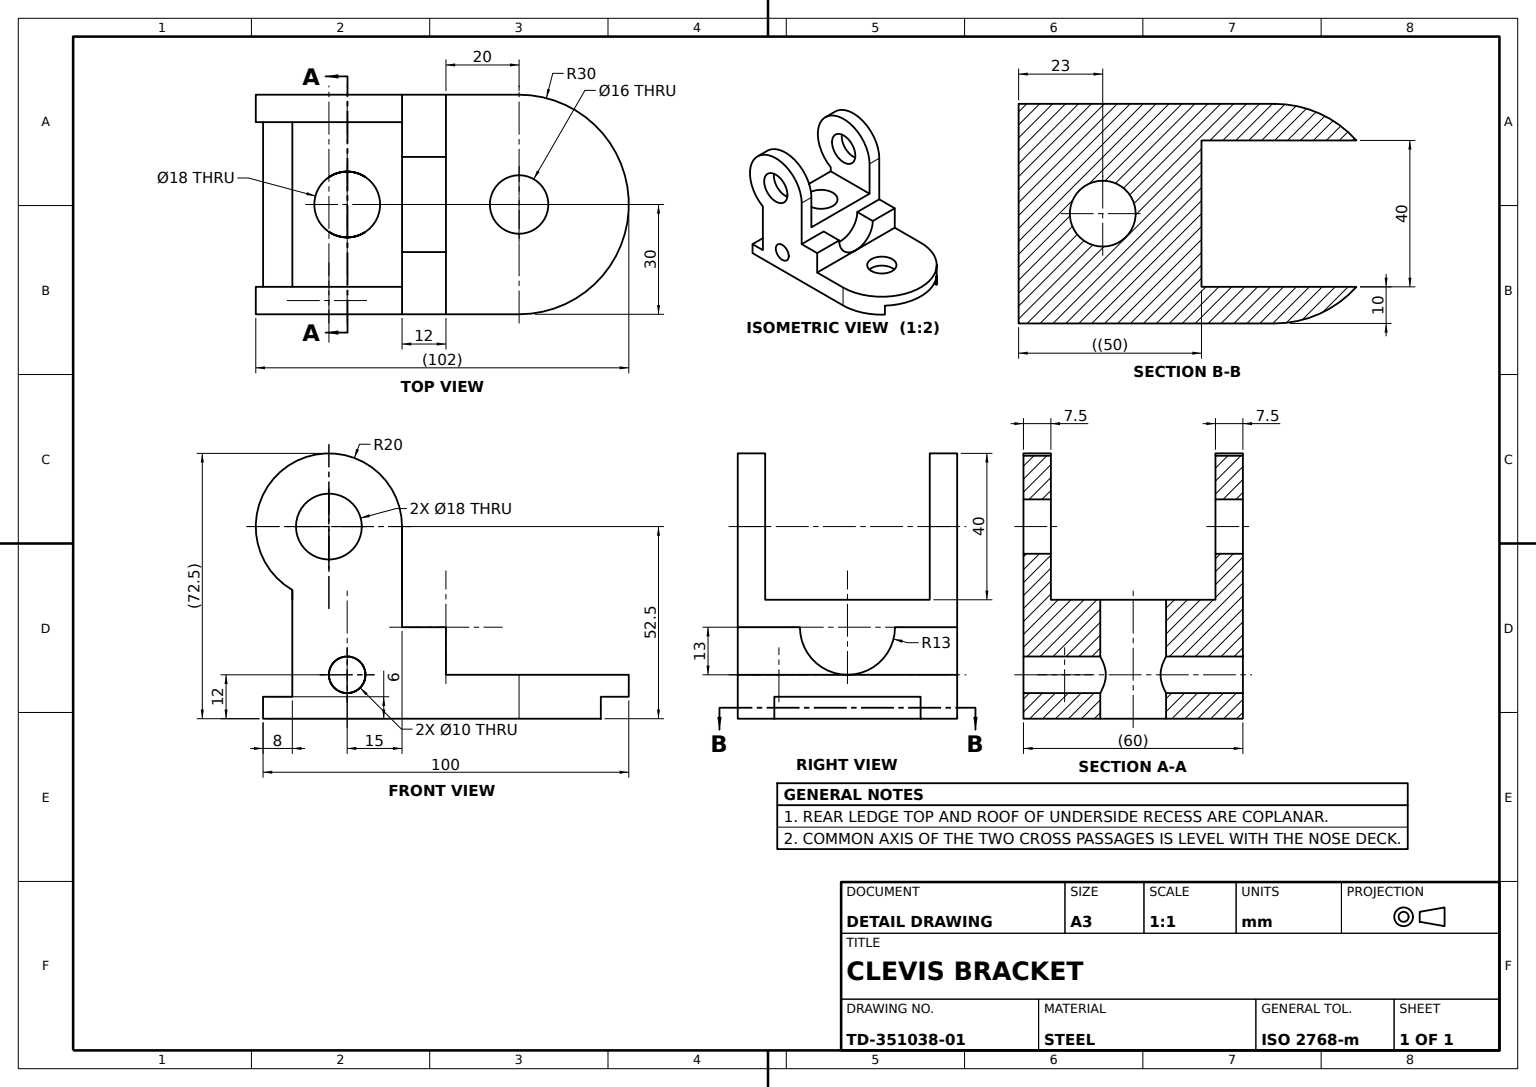
ISO-10303-21;
HEADER;
FILE_DESCRIPTION((''),'2;1');
FILE_NAME('','',(''),(''),'','','');
FILE_SCHEMA(('AUTOMOTIVE_DESIGN'));
ENDSEC;
DATA;
#1=APPLICATION_CONTEXT('');
#2=PRODUCT_CONTEXT('',#1,'mechanical');
#3=PRODUCT('','','',(#2));
#4=PRODUCT_DEFINITION_FORMATION('','',#3);
#5=PRODUCT_DEFINITION_CONTEXT('',#1,'design');
#6=PRODUCT_DEFINITION('','',#4,#5);
#7=PRODUCT_DEFINITION_SHAPE('','',#6);
#8=(LENGTH_UNIT()NAMED_UNIT(*)SI_UNIT(.MILLI.,.METRE.));
#9=(NAMED_UNIT(*)PLANE_ANGLE_UNIT()SI_UNIT($,.RADIAN.));
#10=(NAMED_UNIT(*)SI_UNIT($,.STERADIAN.)SOLID_ANGLE_UNIT());
#11=UNCERTAINTY_MEASURE_WITH_UNIT(LENGTH_MEASURE(1.E-05),#8,'distance_accuracy_value','');
#12=(GEOMETRIC_REPRESENTATION_CONTEXT(3)GLOBAL_UNCERTAINTY_ASSIGNED_CONTEXT((#11))GLOBAL_UNIT_ASSIGNED_CONTEXT((#8,#9,#10))REPRESENTATION_CONTEXT('',''));
#13=CARTESIAN_POINT('',(-13.,25.,-12.));
#14=VERTEX_POINT('',#13);
#15=CARTESIAN_POINT('',(13.,25.,-12.));
#16=VERTEX_POINT('',#15);
#17=CARTESIAN_POINT('',(0.,25.,-12.));
#18=DIRECTION('',(0.,0.,1.));
#19=DIRECTION('',(-1.,0.,0.));
#20=AXIS2_PLACEMENT_3D('',#17,#18,#19);
#21=CIRCLE('',#20,13.);
#22=EDGE_CURVE('',#14,#16,#21,.T.);
#23=ORIENTED_EDGE('',*,*,#22,.F.);
#24=CARTESIAN_POINT('',(-13.,25.,0.));
#25=VERTEX_POINT('',#24);
#26=CARTESIAN_POINT('',(-13.,25.,-41.068884));
#27=VECTOR('',#18,1000.);
#28=LINE('',#26,#27);
#29=EDGE_CURVE('',#14,#25,#28,.T.);
#30=ORIENTED_EDGE('',*,*,#29,.T.);
#31=CARTESIAN_POINT('',(0.,12.,0.));
#32=VERTEX_POINT('',#31);
#33=CARTESIAN_POINT('',(0.,25.,0.));
#34=DIRECTION('',(1.,0.,0.));
#35=AXIS2_PLACEMENT_3D('',#33,#18,#34);
#36=CIRCLE('',#35,13.);
#37=EDGE_CURVE('',#25,#32,#36,.T.);
#38=ORIENTED_EDGE('',*,*,#37,.T.);
#39=CARTESIAN_POINT('',(13.,25.,0.));
#40=VERTEX_POINT('',#39);
#41=EDGE_CURVE('',#32,#40,#36,.T.);
#42=ORIENTED_EDGE('',*,*,#41,.T.);
#43=CARTESIAN_POINT('',(13.,25.,-41.068884));
#44=LINE('',#43,#27);
#45=EDGE_CURVE('',#16,#40,#44,.T.);
#46=ORIENTED_EDGE('',*,*,#45,.F.);
#47=EDGE_LOOP('',(#23,#30,#38,#42,#46));
#48=FACE_OUTER_BOUND('',#47,.T.);
#49=CARTESIAN_POINT('',(0.,25.,-41.068884));
#50=AXIS2_PLACEMENT_3D('',#49,#18,#34);
#51=CYLINDRICAL_SURFACE('',#50,13.);
#52=ADVANCED_FACE('',(#48),#51,.F.);
#53=CARTESIAN_POINT('',(-9.,32.5,-27.));
#54=VERTEX_POINT('',#53);
#55=CARTESIAN_POINT('',(9.,32.5,-27.));
#56=VERTEX_POINT('',#55);
#57=CARTESIAN_POINT('',(0.,32.5,-27.));
#58=DIRECTION('',(0.,1.,0.));
#59=AXIS2_PLACEMENT_3D('',#57,#58,#19);
#60=CIRCLE('',#59,9.);
#61=EDGE_CURVE('',#54,#56,#60,.T.);
#62=ORIENTED_EDGE('',*,*,#61,.T.);
#63=CARTESIAN_POINT('',(9.,17.,-27.));
#64=VERTEX_POINT('',#63);
#65=CARTESIAN_POINT('',(9.,-25.455844,-27.));
#66=VECTOR('',#58,1000.);
#67=LINE('',#65,#66);
#68=EDGE_CURVE('',#64,#56,#67,.T.);
#69=ORIENTED_EDGE('',*,*,#68,.F.);
#70=CARTESIAN_POINT('',(7.483315,12.,-22.));
#71=VERTEX_POINT('',#70);
#72=CARTESIAN_POINT('',(9.,17.,-26.667217));
#73=CARTESIAN_POINT('',(8.980863,16.965779,-26.328396));
#74=CARTESIAN_POINT('',(8.908433,16.833553,-25.67834));
#75=CARTESIAN_POINT('',(8.855396,16.736031,-25.363152));
#76=CARTESIAN_POINT('',(8.720807,16.479333,-24.753929));
#77=CARTESIAN_POINT('',(8.641395,16.324189,-24.469129));
#78=CARTESIAN_POINT('',(8.46662,15.963402,-23.934815));
#79=CARTESIAN_POINT('',(8.370403,15.755736,-23.683896));
#80=CARTESIAN_POINT('',(8.177309,15.303073,-23.232798));
#81=CARTESIAN_POINT('',(8.079797,15.057097,-23.030379));
#82=CARTESIAN_POINT('',(7.939748,14.656179,-22.76082));
#83=CARTESIAN_POINT('',(7.894002,14.516672,-22.676521));
#84=CARTESIAN_POINT('',(7.807992,14.232287,-22.523059));
#85=CARTESIAN_POINT('',(7.767486,14.086776,-22.45341));
#86=CARTESIAN_POINT('',(7.65546,13.639895,-22.265532));
#87=CARTESIAN_POINT('',(7.593346,13.328311,-22.168079));
#88=CARTESIAN_POINT('',(7.506483,12.672902,-22.03421));
#89=CARTESIAN_POINT('',(7.483315,12.337194,-22.));
#90=B_SPLINE_CURVE_WITH_KNOTS('',3,(#63,#72,#73,#74,#75,#76,#77,#78,#79,#80,#81,#82,#83,#84,#85,#86,#87,#88,#89,#70),.UNSPECIFIED.,.F.,.F.,(4,2,2,2,2,2,2,2,2,4),(0.023949869,0.024944888,0.025939907,0.026934926,0.027929944,0.028924963,0.029422472,0.029919982,0.030915,0.031910019),.UNSPECIFIED.);
#91=EDGE_CURVE('',#64,#71,#90,.T.);
#92=ORIENTED_EDGE('',*,*,#91,.T.);
#93=CARTESIAN_POINT('',(9.,7.,-27.));
#94=VERTEX_POINT('',#93);
#95=CARTESIAN_POINT('',(7.483315,11.661464,-22.));
#96=CARTESIAN_POINT('',(7.506333,11.330449,-22.034004));
#97=CARTESIAN_POINT('',(7.59168,10.682097,-22.165484));
#98=CARTESIAN_POINT('',(7.654971,10.361958,-22.264699));
#99=CARTESIAN_POINT('',(7.805667,9.761018,-22.517454));
#100=CARTESIAN_POINT('',(7.893121,9.477151,-22.671007));
#101=CARTESIAN_POINT('',(8.08099,8.93964,-23.032742));
#102=CARTESIAN_POINT('',(8.179185,8.692305,-23.236859));
#103=CARTESIAN_POINT('',(8.323959,8.353256,-23.575562));
#104=CARTESIAN_POINT('',(8.37188,8.245445,-23.69405));
#105=CARTESIAN_POINT('',(8.465872,8.040291,-23.942764));
#106=CARTESIAN_POINT('',(8.512072,7.94271,-24.073476));
#107=CARTESIAN_POINT('',(8.643395,7.671811,-24.475847));
#108=CARTESIAN_POINT('',(8.72219,7.518012,-24.759837));
#109=CARTESIAN_POINT('',(8.854968,7.264805,-25.361564));
#110=CARTESIAN_POINT('',(8.909233,7.164975,-25.68371));
#111=CARTESIAN_POINT('',(8.981296,7.033441,-26.334133));
#112=CARTESIAN_POINT('',(9.,7.,-26.664417));
#113=B_SPLINE_CURVE_WITH_KNOTS('',3,(#70,#95,#96,#97,#98,#99,#100,#101,#102,#103,#104,#105,#106,#107,#108,#109,#110,#111,#112,#93),.UNSPECIFIED.,.F.,.F.,(4,2,2,2,2,2,2,2,2,4),(0.,0.000998979,0.001997959,0.002996938,0.003995917,0.004495407,0.004994896,0.005993876,0.006992855,0.007991834),.UNSPECIFIED.);
#114=EDGE_CURVE('',#71,#94,#113,.T.);
#115=ORIENTED_EDGE('',*,*,#114,.T.);
#116=CARTESIAN_POINT('',(9.,0.,-27.));
#117=VERTEX_POINT('',#116);
#118=EDGE_CURVE('',#117,#94,#67,.T.);
#119=ORIENTED_EDGE('',*,*,#118,.F.);
#120=CARTESIAN_POINT('',(-9.,0.,-27.));
#121=VERTEX_POINT('',#120);
#122=CARTESIAN_POINT('',(0.,0.,-27.));
#123=DIRECTION('',(0.,-1.,0.));
#124=AXIS2_PLACEMENT_3D('',#122,#123,#18);
#125=CIRCLE('',#124,9.);
#126=EDGE_CURVE('',#117,#121,#125,.T.);
#127=ORIENTED_EDGE('',*,*,#126,.T.);
#128=CARTESIAN_POINT('',(-9.,7.,-27.));
#129=VERTEX_POINT('',#128);
#130=CARTESIAN_POINT('',(-9.,-25.455844,-27.));
#131=LINE('',#130,#66);
#132=EDGE_CURVE('',#121,#129,#131,.T.);
#133=ORIENTED_EDGE('',*,*,#132,.T.);
#134=CARTESIAN_POINT('',(-7.483315,12.,-22.));
#135=VERTEX_POINT('',#134);
#136=CARTESIAN_POINT('',(-9.,7.,-26.667217));
#137=CARTESIAN_POINT('',(-8.980863,7.034221,-26.328396));
#138=CARTESIAN_POINT('',(-8.908433,7.166447,-25.67834));
#139=CARTESIAN_POINT('',(-8.855396,7.263969,-25.363152));
#140=CARTESIAN_POINT('',(-8.720807,7.520667,-24.753929));
#141=CARTESIAN_POINT('',(-8.641395,7.675811,-24.469129));
#142=CARTESIAN_POINT('',(-8.46662,8.036598,-23.934815));
#143=CARTESIAN_POINT('',(-8.370403,8.244264,-23.683896));
#144=CARTESIAN_POINT('',(-8.177309,8.696927,-23.232798));
#145=CARTESIAN_POINT('',(-8.079797,8.942903,-23.030379));
#146=CARTESIAN_POINT('',(-7.939748,9.343821,-22.76082));
#147=CARTESIAN_POINT('',(-7.894002,9.483328,-22.676521));
#148=CARTESIAN_POINT('',(-7.807992,9.767713,-22.523059));
#149=CARTESIAN_POINT('',(-7.767486,9.913224,-22.45341));
#150=CARTESIAN_POINT('',(-7.65546,10.360105,-22.265532));
#151=CARTESIAN_POINT('',(-7.593346,10.671689,-22.168079));
#152=CARTESIAN_POINT('',(-7.506483,11.327098,-22.03421));
#153=CARTESIAN_POINT('',(-7.483315,11.662806,-22.));
#154=B_SPLINE_CURVE_WITH_KNOTS('',3,(#128,#136,#137,#138,#139,#140,#141,#142,#143,#144,#145,#146,#147,#148,#149,#150,#151,#152,#153,#134),.UNSPECIFIED.,.F.,.F.,(4,2,2,2,2,2,2,2,2,4),(0.023949869,0.024944888,0.025939907,0.026934926,0.027929944,0.028924963,0.029422472,0.029919982,0.030915,0.031910019),.UNSPECIFIED.);
#155=EDGE_CURVE('',#129,#135,#154,.T.);
#156=ORIENTED_EDGE('',*,*,#155,.T.);
#157=CARTESIAN_POINT('',(-9.,17.,-27.));
#158=VERTEX_POINT('',#157);
#159=CARTESIAN_POINT('',(-7.483315,12.338536,-22.));
#160=CARTESIAN_POINT('',(-7.506333,12.669551,-22.034004));
#161=CARTESIAN_POINT('',(-7.59168,13.317903,-22.165484));
#162=CARTESIAN_POINT('',(-7.654971,13.638042,-22.264699));
#163=CARTESIAN_POINT('',(-7.805667,14.238982,-22.517454));
#164=CARTESIAN_POINT('',(-7.893121,14.522849,-22.671007));
#165=CARTESIAN_POINT('',(-8.08099,15.06036,-23.032742));
#166=CARTESIAN_POINT('',(-8.179185,15.307695,-23.236859));
#167=CARTESIAN_POINT('',(-8.323959,15.646744,-23.575562));
#168=CARTESIAN_POINT('',(-8.37188,15.754555,-23.69405));
#169=CARTESIAN_POINT('',(-8.465872,15.959709,-23.942764));
#170=CARTESIAN_POINT('',(-8.512072,16.05729,-24.073476));
#171=CARTESIAN_POINT('',(-8.643395,16.328189,-24.475847));
#172=CARTESIAN_POINT('',(-8.72219,16.481988,-24.759837));
#173=CARTESIAN_POINT('',(-8.854968,16.735195,-25.361564));
#174=CARTESIAN_POINT('',(-8.909233,16.835025,-25.68371));
#175=CARTESIAN_POINT('',(-8.981296,16.966559,-26.334133));
#176=CARTESIAN_POINT('',(-9.,17.,-26.664417));
#177=B_SPLINE_CURVE_WITH_KNOTS('',3,(#134,#159,#160,#161,#162,#163,#164,#165,#166,#167,#168,#169,#170,#171,#172,#173,#174,#175,#176,#157),.UNSPECIFIED.,.F.,.F.,(4,2,2,2,2,2,2,2,2,4),(0.,0.000998979,0.001997959,0.002996938,0.003995917,0.004495407,0.004994896,0.005993876,0.006992855,0.007991834),.UNSPECIFIED.);
#178=EDGE_CURVE('',#135,#158,#177,.T.);
#179=ORIENTED_EDGE('',*,*,#178,.T.);
#180=EDGE_CURVE('',#158,#54,#131,.T.);
#181=ORIENTED_EDGE('',*,*,#180,.T.);
#182=EDGE_LOOP('',(#62,#69,#92,#115,#119,#127,#133,#156,#179,#181));
#183=FACE_OUTER_BOUND('',#182,.T.);
#184=CARTESIAN_POINT('',(0.,-25.455844,-27.));
#185=AXIS2_PLACEMENT_3D('',#184,#58,#19);
#186=CYLINDRICAL_SURFACE('',#185,9.);
#187=ADVANCED_FACE('',(#183),#186,.F.);
#188=CARTESIAN_POINT('',(30.,12.,-22.));
#189=VERTEX_POINT('',#188);
#190=VECTOR('',#19,1000.);
#191=LINE('',#188,#190);
#192=EDGE_CURVE('',#189,#71,#191,.T.);
#193=ORIENTED_EDGE('',*,*,#192,.F.);
#194=CARTESIAN_POINT('',(30.,12.,-32.));
#195=VERTEX_POINT('',#194);
#196=CARTESIAN_POINT('',(30.,12.,-27.));
#197=DIRECTION('',(0.,0.,-1.));
#198=AXIS2_PLACEMENT_3D('',#196,#34,#197);
#199=CIRCLE('',#198,5.);
#200=EDGE_CURVE('',#189,#195,#199,.T.);
#201=ORIENTED_EDGE('',*,*,#200,.T.);
#202=CARTESIAN_POINT('',(7.483315,12.,-32.));
#203=VERTEX_POINT('',#202);
#204=LINE('',#194,#190);
#205=EDGE_CURVE('',#195,#203,#204,.T.);
#206=ORIENTED_EDGE('',*,*,#205,.T.);
#207=CARTESIAN_POINT('',(9.,7.,-27.167631));
#208=CARTESIAN_POINT('',(8.995223,7.008583,-27.337323));
#209=CARTESIAN_POINT('',(8.976544,7.042326,-27.670444));
#210=CARTESIAN_POINT('',(8.962682,7.067412,-27.83489));
#211=CARTESIAN_POINT('',(8.926465,7.133529,-28.15971));
#212=CARTESIAN_POINT('',(8.904109,7.174561,-28.320084));
#213=CARTESIAN_POINT('',(8.851364,7.272595,-28.636804));
#214=CARTESIAN_POINT('',(8.820832,7.329878,-28.793592));
#215=CARTESIAN_POINT('',(8.720282,7.521699,-29.247864));
#216=CARTESIAN_POINT('',(8.640877,7.676808,-29.532795));
#217=CARTESIAN_POINT('',(8.465025,8.039964,-30.069716));
#218=CARTESIAN_POINT('',(8.369097,8.24717,-30.319378));
#219=CARTESIAN_POINT('',(8.176067,8.699998,-30.769879));
#220=CARTESIAN_POINT('',(8.077598,8.948613,-30.974109));
#221=CARTESIAN_POINT('',(7.890372,9.485772,-31.333955));
#222=CARTESIAN_POINT('',(7.803491,9.768824,-31.486288));
#223=CARTESIAN_POINT('',(7.691444,10.21696,-31.674078));
#224=CARTESIAN_POINT('',(7.657154,10.370296,-31.729829));
#225=CARTESIAN_POINT('',(7.596294,10.685616,-31.826967));
#226=CARTESIAN_POINT('',(7.569684,10.848409,-31.868411));
#227=CARTESIAN_POINT('',(7.505701,11.336851,-31.966949));
#228=CARTESIAN_POINT('',(7.483315,11.666392,-32.));
#229=B_SPLINE_CURVE_WITH_KNOTS('',3,(#93,#207,#208,#209,#210,#211,#212,#213,#214,#215,#216,#217,#218,#219,#220,#221,#222,#223,#224,#225,#226,#227,#228,#202),.UNSPECIFIED.,.F.,.F.,(4,2,2,2,2,2,2,2,2,2,2,4),(0.007991834,0.008490847,0.00898986,0.009488874,0.009987887,0.010985913,0.011983939,0.012981966,0.013979992,0.014479005,0.014978018,0.015976045),.UNSPECIFIED.);
#230=EDGE_CURVE('',#94,#203,#229,.T.);
#231=ORIENTED_EDGE('',*,*,#230,.F.);
#232=ORIENTED_EDGE('',*,*,#114,.F.);
#233=EDGE_LOOP('',(#193,#201,#206,#231,#232));
#234=FACE_OUTER_BOUND('',#233,.T.);
#235=AXIS2_PLACEMENT_3D('',#196,#19,#18);
#236=CYLINDRICAL_SURFACE('',#235,5.);
#237=ADVANCED_FACE('',(#234),#236,.F.);
#238=CARTESIAN_POINT('',(20.,6.,0.));
#239=VERTEX_POINT('',#238);
#240=CARTESIAN_POINT('',(-20.,6.,0.));
#241=VERTEX_POINT('',#240);
#242=LINE('',#240,#190);
#243=EDGE_CURVE('',#239,#241,#242,.T.);
#244=ORIENTED_EDGE('',*,*,#243,.F.);
#245=CARTESIAN_POINT('',(20.,6.,42.36068));
#246=VERTEX_POINT('',#245);
#247=CARTESIAN_POINT('',(20.,6.,50.001));
#248=VECTOR('',#197,1000.);
#249=LINE('',#247,#248);
#250=EDGE_CURVE('',#246,#239,#249,.T.);
#251=ORIENTED_EDGE('',*,*,#250,.F.);
#252=CARTESIAN_POINT('',(-20.,6.,42.36068));
#253=VERTEX_POINT('',#252);
#254=CARTESIAN_POINT('',(0.,6.,20.));
#255=AXIS2_PLACEMENT_3D('',#254,#123,#197);
#256=CIRCLE('',#255,30.);
#257=EDGE_CURVE('',#246,#253,#256,.T.);
#258=ORIENTED_EDGE('',*,*,#257,.T.);
#259=CARTESIAN_POINT('',(-20.,6.,50.001));
#260=LINE('',#259,#248);
#261=EDGE_CURVE('',#253,#241,#260,.T.);
#262=ORIENTED_EDGE('',*,*,#261,.T.);
#263=EDGE_LOOP('',(#244,#251,#258,#262));
#264=FACE_OUTER_BOUND('',#263,.T.);
#265=CARTESIAN_POINT('',(-8.,6.,20.));
#266=VERTEX_POINT('',#265);
#267=CARTESIAN_POINT('',(8.,6.,20.));
#268=VERTEX_POINT('',#267);
#269=CIRCLE('',#255,8.);
#270=EDGE_CURVE('',#266,#268,#269,.T.);
#271=ORIENTED_EDGE('',*,*,#270,.F.);
#272=EDGE_CURVE('',#268,#266,#269,.T.);
#273=ORIENTED_EDGE('',*,*,#272,.F.);
#274=EDGE_LOOP('',(#271,#273));
#275=FACE_BOUND('',#274,.T.);
#276=AXIS2_PLACEMENT_3D('',#259,#123,#197);
#277=PLANE('',#276);
#278=ADVANCED_FACE('',(#264,#275),#277,.T.);
#279=CARTESIAN_POINT('',(30.,12.,0.));
#280=VERTEX_POINT('',#279);
#281=CARTESIAN_POINT('',(30.,12.,20.));
#282=VERTEX_POINT('',#281);
#283=CARTESIAN_POINT('',(30.,12.,50.));
#284=LINE('',#283,#27);
#285=EDGE_CURVE('',#280,#282,#284,.T.);
#286=ORIENTED_EDGE('',*,*,#285,.F.);
#287=LINE('',#279,#190);
#288=EDGE_CURVE('',#280,#32,#287,.T.);
#289=ORIENTED_EDGE('',*,*,#288,.T.);
#290=CARTESIAN_POINT('',(-30.,12.,0.));
#291=VERTEX_POINT('',#290);
#292=EDGE_CURVE('',#32,#291,#287,.T.);
#293=ORIENTED_EDGE('',*,*,#292,.T.);
#294=CARTESIAN_POINT('',(-30.,12.,20.));
#295=VERTEX_POINT('',#294);
#296=CARTESIAN_POINT('',(-30.,12.,50.));
#297=LINE('',#296,#27);
#298=EDGE_CURVE('',#291,#295,#297,.T.);
#299=ORIENTED_EDGE('',*,*,#298,.T.);
#300=CARTESIAN_POINT('',(0.,12.,20.));
#301=AXIS2_PLACEMENT_3D('',#300,#58,#197);
#302=CIRCLE('',#301,30.);
#303=EDGE_CURVE('',#295,#282,#302,.T.);
#304=ORIENTED_EDGE('',*,*,#303,.T.);
#305=EDGE_LOOP('',(#286,#289,#293,#299,#304));
#306=FACE_OUTER_BOUND('',#305,.T.);
#307=CARTESIAN_POINT('',(8.,12.,20.));
#308=VERTEX_POINT('',#307);
#309=CARTESIAN_POINT('',(-8.,12.,20.));
#310=VERTEX_POINT('',#309);
#311=AXIS2_PLACEMENT_3D('',#300,#123,#197);
#312=CIRCLE('',#311,8.);
#313=EDGE_CURVE('',#308,#310,#312,.T.);
#314=ORIENTED_EDGE('',*,*,#313,.T.);
#315=EDGE_CURVE('',#310,#308,#312,.T.);
#316=ORIENTED_EDGE('',*,*,#315,.T.);
#317=EDGE_LOOP('',(#314,#316));
#318=FACE_BOUND('',#317,.T.);
#319=AXIS2_PLACEMENT_3D('',#283,#123,#197);
#320=PLANE('',#319);
#321=ADVANCED_FACE('',(#306,#318),#320,.F.);
#322=CARTESIAN_POINT('',(22.5,52.5,-41.));
#323=VERTEX_POINT('',#322);
#324=CARTESIAN_POINT('',(22.5,52.5,-23.));
#325=VERTEX_POINT('',#324);
#326=CARTESIAN_POINT('',(22.5,52.5,-32.));
#327=AXIS2_PLACEMENT_3D('',#326,#19,#58);
#328=CIRCLE('',#327,9.);
#329=EDGE_CURVE('',#323,#325,#328,.T.);
#330=ORIENTED_EDGE('',*,*,#329,.F.);
#331=EDGE_CURVE('',#325,#323,#328,.T.);
#332=ORIENTED_EDGE('',*,*,#331,.F.);
#333=EDGE_LOOP('',(#330,#332));
#334=FACE_BOUND('',#333,.T.);
#335=CARTESIAN_POINT('',(22.5,32.5,-42.));
#336=VERTEX_POINT('',#335);
#337=CARTESIAN_POINT('',(22.5,32.5,-12.));
#338=VERTEX_POINT('',#337);
#339=CARTESIAN_POINT('',(22.5,32.5,-52.001));
#340=LINE('',#339,#27);
#341=EDGE_CURVE('',#336,#338,#340,.T.);
#342=ORIENTED_EDGE('',*,*,#341,.T.);
#343=CARTESIAN_POINT('',(22.5,52.5,-12.));
#344=VERTEX_POINT('',#343);
#345=CARTESIAN_POINT('',(22.5,72.5,-12.));
#346=LINE('',#345,#66);
#347=EDGE_CURVE('',#338,#344,#346,.T.);
#348=ORIENTED_EDGE('',*,*,#347,.T.);
#349=CARTESIAN_POINT('',(22.5,35.179492,-42.));
#350=VERTEX_POINT('',#349);
#351=CIRCLE('',#327,20.);
#352=EDGE_CURVE('',#344,#350,#351,.T.);
#353=ORIENTED_EDGE('',*,*,#352,.T.);
#354=CARTESIAN_POINT('',(22.5,72.5,-42.));
#355=VECTOR('',#123,1000.);
#356=LINE('',#354,#355);
#357=EDGE_CURVE('',#350,#336,#356,.T.);
#358=ORIENTED_EDGE('',*,*,#357,.T.);
#359=EDGE_LOOP('',(#342,#348,#353,#358));
#360=FACE_OUTER_BOUND('',#359,.T.);
#361=CARTESIAN_POINT('',(22.5,72.5,-52.001));
#362=AXIS2_PLACEMENT_3D('',#361,#34,#58);
#363=PLANE('',#362);
#364=ADVANCED_FACE('',(#334,#360),#363,.F.);
#365=CARTESIAN_POINT('',(-22.5,52.5,-23.));
#366=VERTEX_POINT('',#365);
#367=CARTESIAN_POINT('',(-30.,52.5,-23.));
#368=VERTEX_POINT('',#367);
#369=CARTESIAN_POINT('',(30.,52.5,-23.));
#370=LINE('',#369,#190);
#371=EDGE_CURVE('',#366,#368,#370,.T.);
#372=ORIENTED_EDGE('',*,*,#371,.T.);
#373=CARTESIAN_POINT('',(-30.,52.5,-41.));
#374=VERTEX_POINT('',#373);
#375=CARTESIAN_POINT('',(-30.,52.5,-32.));
#376=AXIS2_PLACEMENT_3D('',#375,#34,#197);
#377=CIRCLE('',#376,9.);
#378=EDGE_CURVE('',#374,#368,#377,.T.);
#379=ORIENTED_EDGE('',*,*,#378,.F.);
#380=CARTESIAN_POINT('',(-22.5,52.5,-41.));
#381=VERTEX_POINT('',#380);
#382=CARTESIAN_POINT('',(30.,52.5,-41.));
#383=LINE('',#382,#190);
#384=EDGE_CURVE('',#381,#374,#383,.T.);
#385=ORIENTED_EDGE('',*,*,#384,.F.);
#386=CARTESIAN_POINT('',(-22.5,52.5,-32.));
#387=AXIS2_PLACEMENT_3D('',#386,#34,#123);
#388=CIRCLE('',#387,9.);
#389=EDGE_CURVE('',#381,#366,#388,.T.);
#390=ORIENTED_EDGE('',*,*,#389,.T.);
#391=EDGE_LOOP('',(#372,#379,#385,#390));
#392=FACE_OUTER_BOUND('',#391,.T.);
#393=CARTESIAN_POINT('',(30.,52.5,-32.));
#394=AXIS2_PLACEMENT_3D('',#393,#19,#18);
#395=CYLINDRICAL_SURFACE('',#394,9.);
#396=ADVANCED_FACE('',(#392),#395,.F.);
#397=ORIENTED_EDGE('',*,*,#261,.F.);
#398=CARTESIAN_POINT('',(-20.,0.,42.36068));
#399=VERTEX_POINT('',#398);
#400=LINE('',#398,#355);
#401=EDGE_CURVE('',#253,#399,#400,.T.);
#402=ORIENTED_EDGE('',*,*,#401,.T.);
#403=CARTESIAN_POINT('',(-20.,0.,0.));
#404=VERTEX_POINT('',#403);
#405=CARTESIAN_POINT('',(-20.,0.,50.001));
#406=LINE('',#405,#248);
#407=EDGE_CURVE('',#399,#404,#406,.T.);
#408=ORIENTED_EDGE('',*,*,#407,.T.);
#409=LINE('',#403,#355);
#410=EDGE_CURVE('',#241,#404,#409,.T.);
#411=ORIENTED_EDGE('',*,*,#410,.F.);
#412=EDGE_LOOP('',(#397,#402,#408,#411));
#413=FACE_OUTER_BOUND('',#412,.T.);
#414=AXIS2_PLACEMENT_3D('',#405,#34,#197);
#415=PLANE('',#414);
#416=ADVANCED_FACE('',(#413),#415,.T.);
#417=CARTESIAN_POINT('',(30.,6.,-50.));
#418=VERTEX_POINT('',#417);
#419=CARTESIAN_POINT('',(-30.,6.,-50.));
#420=VERTEX_POINT('',#419);
#421=LINE('',#417,#190);
#422=EDGE_CURVE('',#418,#420,#421,.T.);
#423=ORIENTED_EDGE('',*,*,#422,.F.);
#424=CARTESIAN_POINT('',(30.,0.,-50.));
#425=VERTEX_POINT('',#424);
#426=LINE('',#424,#66);
#427=EDGE_CURVE('',#425,#418,#426,.T.);
#428=ORIENTED_EDGE('',*,*,#427,.F.);
#429=CARTESIAN_POINT('',(-30.,0.,-50.));
#430=VERTEX_POINT('',#429);
#431=LINE('',#424,#190);
#432=EDGE_CURVE('',#425,#430,#431,.T.);
#433=ORIENTED_EDGE('',*,*,#432,.T.);
#434=LINE('',#429,#66);
#435=EDGE_CURVE('',#430,#420,#434,.T.);
#436=ORIENTED_EDGE('',*,*,#435,.T.);
#437=EDGE_LOOP('',(#423,#428,#433,#436));
#438=FACE_OUTER_BOUND('',#437,.T.);
#439=AXIS2_PLACEMENT_3D('',#424,#18,#34);
#440=PLANE('',#439);
#441=ADVANCED_FACE('',(#438),#440,.F.);
#442=ORIENTED_EDGE('',*,*,#329,.T.);
#443=VERTEX_POINT('',#369);
#444=EDGE_CURVE('',#443,#325,#370,.T.);
#445=ORIENTED_EDGE('',*,*,#444,.F.);
#446=VERTEX_POINT('',#382);
#447=AXIS2_PLACEMENT_3D('',#393,#34,#197);
#448=CIRCLE('',#447,9.);
#449=EDGE_CURVE('',#443,#446,#448,.T.);
#450=ORIENTED_EDGE('',*,*,#449,.T.);
#451=EDGE_CURVE('',#446,#323,#383,.T.);
#452=ORIENTED_EDGE('',*,*,#451,.T.);
#453=EDGE_LOOP('',(#442,#445,#450,#452));
#454=FACE_OUTER_BOUND('',#453,.T.);
#455=ADVANCED_FACE('',(#454),#395,.F.);
#456=CARTESIAN_POINT('',(-30.,35.179492,-42.));
#457=VERTEX_POINT('',#456);
#458=CARTESIAN_POINT('',(-30.,52.5,-12.));
#459=VERTEX_POINT('',#458);
#460=CIRCLE('',#376,20.);
#461=EDGE_CURVE('',#457,#459,#460,.T.);
#462=ORIENTED_EDGE('',*,*,#461,.F.);
#463=CARTESIAN_POINT('',(-30.,6.,-42.));
#464=VERTEX_POINT('',#463);
#465=LINE('',#463,#66);
#466=EDGE_CURVE('',#464,#457,#465,.T.);
#467=ORIENTED_EDGE('',*,*,#466,.F.);
#468=LINE('',#419,#27);
#469=EDGE_CURVE('',#420,#464,#468,.T.);
#470=ORIENTED_EDGE('',*,*,#469,.F.);
#471=ORIENTED_EDGE('',*,*,#435,.F.);
#472=CARTESIAN_POINT('',(-30.,0.,20.));
#473=VERTEX_POINT('',#472);
#474=CARTESIAN_POINT('',(-30.,0.,50.));
#475=LINE('',#474,#248);
#476=EDGE_CURVE('',#473,#430,#475,.T.);
#477=ORIENTED_EDGE('',*,*,#476,.F.);
#478=CARTESIAN_POINT('',(-30.,52.5,20.));
#479=LINE('',#478,#66);
#480=EDGE_CURVE('',#473,#295,#479,.T.);
#481=ORIENTED_EDGE('',*,*,#480,.T.);
#482=ORIENTED_EDGE('',*,*,#298,.F.);
#483=CARTESIAN_POINT('',(-30.,25.,0.));
#484=VERTEX_POINT('',#483);
#485=LINE('',#290,#355);
#486=EDGE_CURVE('',#484,#291,#485,.T.);
#487=ORIENTED_EDGE('',*,*,#486,.F.);
#488=CARTESIAN_POINT('',(-30.,25.,-12.));
#489=VERTEX_POINT('',#488);
#490=LINE('',#483,#27);
#491=EDGE_CURVE('',#489,#484,#490,.T.);
#492=ORIENTED_EDGE('',*,*,#491,.F.);
#493=LINE('',#488,#355);
#494=EDGE_CURVE('',#459,#489,#493,.T.);
#495=ORIENTED_EDGE('',*,*,#494,.F.);
#496=EDGE_LOOP('',(#462,#467,#470,#471,#477,#481,#482,#487,#492,#495));
#497=FACE_OUTER_BOUND('',#496,.T.);
#498=CARTESIAN_POINT('',(-30.,12.,-22.));
#499=VERTEX_POINT('',#498);
#500=CARTESIAN_POINT('',(-30.,12.,-32.));
#501=VERTEX_POINT('',#500);
#502=CARTESIAN_POINT('',(-30.,12.,-27.));
#503=AXIS2_PLACEMENT_3D('',#502,#34,#197);
#504=CIRCLE('',#503,5.);
#505=EDGE_CURVE('',#499,#501,#504,.T.);
#506=ORIENTED_EDGE('',*,*,#505,.T.);
#507=EDGE_CURVE('',#501,#499,#504,.T.);
#508=ORIENTED_EDGE('',*,*,#507,.T.);
#509=EDGE_LOOP('',(#506,#508));
#510=FACE_BOUND('',#509,.T.);
#511=EDGE_CURVE('',#368,#374,#377,.T.);
#512=ORIENTED_EDGE('',*,*,#511,.T.);
#513=ORIENTED_EDGE('',*,*,#378,.T.);
#514=EDGE_LOOP('',(#512,#513));
#515=FACE_BOUND('',#514,.T.);
#516=PLANE('',#376);
#517=ADVANCED_FACE('',(#497,#510,#515),#516,.F.);
#518=ORIENTED_EDGE('',*,*,#494,.T.);
#519=CARTESIAN_POINT('',(30.,25.,-12.));
#520=LINE('',#519,#190);
#521=EDGE_CURVE('',#14,#489,#520,.T.);
#522=ORIENTED_EDGE('',*,*,#521,.F.);
#523=ORIENTED_EDGE('',*,*,#22,.T.);
#524=VERTEX_POINT('',#519);
#525=EDGE_CURVE('',#524,#16,#520,.T.);
#526=ORIENTED_EDGE('',*,*,#525,.F.);
#527=CARTESIAN_POINT('',(30.,52.5,-12.));
#528=VERTEX_POINT('',#527);
#529=LINE('',#519,#355);
#530=EDGE_CURVE('',#528,#524,#529,.T.);
#531=ORIENTED_EDGE('',*,*,#530,.F.);
#532=LINE('',#527,#190);
#533=EDGE_CURVE('',#528,#344,#532,.T.);
#534=ORIENTED_EDGE('',*,*,#533,.T.);
#535=ORIENTED_EDGE('',*,*,#347,.F.);
#536=CARTESIAN_POINT('',(-22.5,32.5,-12.));
#537=VERTEX_POINT('',#536);
#538=VECTOR('',#34,1000.);
#539=LINE('',#337,#538);
#540=EDGE_CURVE('',#537,#338,#539,.T.);
#541=ORIENTED_EDGE('',*,*,#540,.F.);
#542=CARTESIAN_POINT('',(-22.5,52.5,-12.));
#543=VERTEX_POINT('',#542);
#544=CARTESIAN_POINT('',(-22.5,72.5,-12.));
#545=LINE('',#544,#355);
#546=EDGE_CURVE('',#543,#537,#545,.T.);
#547=ORIENTED_EDGE('',*,*,#546,.F.);
#548=EDGE_CURVE('',#543,#459,#532,.T.);
#549=ORIENTED_EDGE('',*,*,#548,.T.);
#550=EDGE_LOOP('',(#518,#522,#523,#526,#531,#534,#535,#541,#547,#549));
#551=FACE_OUTER_BOUND('',#550,.T.);
#552=AXIS2_PLACEMENT_3D('',#519,#197,#19);
#553=PLANE('',#552);
#554=ADVANCED_FACE('',(#551),#553,.F.);
#555=EDGE_CURVE('',#121,#117,#125,.T.);
#556=ORIENTED_EDGE('',*,*,#555,.T.);
#557=ORIENTED_EDGE('',*,*,#118,.T.);
#558=ORIENTED_EDGE('',*,*,#230,.T.);
#559=CARTESIAN_POINT('',(7.483315,12.333174,-32.));
#560=CARTESIAN_POINT('',(7.506574,12.672339,-31.965636));
#561=CARTESIAN_POINT('',(7.592228,13.321106,-31.833659));
#562=CARTESIAN_POINT('',(7.654905,13.637996,-31.735434));
#563=CARTESIAN_POINT('',(7.80648,14.242007,-31.481158));
#564=CARTESIAN_POINT('',(7.894012,14.525482,-31.327315));
#565=CARTESIAN_POINT('',(8.080802,15.059738,-30.967583));
#566=CARTESIAN_POINT('',(8.180042,15.309793,-30.761272));
#567=CARTESIAN_POINT('',(8.372885,15.761231,-30.30984));
#568=CARTESIAN_POINT('',(8.46746,15.965245,-30.063134));
#569=CARTESIAN_POINT('',(8.643745,16.328928,-29.523161));
#570=CARTESIAN_POINT('',(8.722888,16.483334,-29.237307));
#571=CARTESIAN_POINT('',(8.822049,16.672412,-28.787463));
#572=CARTESIAN_POINT('',(8.851906,16.728418,-28.633794));
#573=CARTESIAN_POINT('',(8.904319,16.825825,-28.31857));
#574=CARTESIAN_POINT('',(8.926991,16.867437,-28.155874));
#575=CARTESIAN_POINT('',(8.981535,16.966996,-27.663994));
#576=CARTESIAN_POINT('',(9.,17.,-27.333355));
#577=B_SPLINE_CURVE_WITH_KNOTS('',3,(#202,#559,#560,#561,#562,#563,#564,#565,#566,#567,#568,#569,#570,#571,#572,#573,#574,#575,#576,#63),.UNSPECIFIED.,.F.,.F.,(4,2,2,2,2,2,2,2,2,4),(0.015976045,0.016972773,0.017969501,0.018966229,0.019962957,0.020959685,0.021956413,0.022454777,0.022953141,0.023949869),.UNSPECIFIED.);
#578=EDGE_CURVE('',#203,#64,#577,.T.);
#579=ORIENTED_EDGE('',*,*,#578,.T.);
#580=ORIENTED_EDGE('',*,*,#68,.T.);
#581=EDGE_CURVE('',#56,#54,#60,.T.);
#582=ORIENTED_EDGE('',*,*,#581,.T.);
#583=ORIENTED_EDGE('',*,*,#180,.F.);
#584=CARTESIAN_POINT('',(-7.483315,12.,-32.));
#585=VERTEX_POINT('',#584);
#586=CARTESIAN_POINT('',(-9.,17.,-27.167631));
#587=CARTESIAN_POINT('',(-8.995223,16.991417,-27.337323));
#588=CARTESIAN_POINT('',(-8.976544,16.957674,-27.670444));
#589=CARTESIAN_POINT('',(-8.962682,16.932588,-27.83489));
#590=CARTESIAN_POINT('',(-8.926465,16.866471,-28.15971));
#591=CARTESIAN_POINT('',(-8.904109,16.825439,-28.320084));
#592=CARTESIAN_POINT('',(-8.851364,16.727405,-28.636804));
#593=CARTESIAN_POINT('',(-8.820832,16.670122,-28.793592));
#594=CARTESIAN_POINT('',(-8.720282,16.478301,-29.247864));
#595=CARTESIAN_POINT('',(-8.640877,16.323192,-29.532795));
#596=CARTESIAN_POINT('',(-8.465025,15.960036,-30.069716));
#597=CARTESIAN_POINT('',(-8.369097,15.75283,-30.319378));
#598=CARTESIAN_POINT('',(-8.176067,15.300002,-30.769879));
#599=CARTESIAN_POINT('',(-8.077598,15.051387,-30.974109));
#600=CARTESIAN_POINT('',(-7.890372,14.514228,-31.333955));
#601=CARTESIAN_POINT('',(-7.803491,14.231176,-31.486288));
#602=CARTESIAN_POINT('',(-7.691444,13.78304,-31.674078));
#603=CARTESIAN_POINT('',(-7.657154,13.629704,-31.729829));
#604=CARTESIAN_POINT('',(-7.596294,13.314384,-31.826967));
#605=CARTESIAN_POINT('',(-7.569684,13.151591,-31.868411));
#606=CARTESIAN_POINT('',(-7.505701,12.663149,-31.966949));
#607=CARTESIAN_POINT('',(-7.483315,12.333608,-32.));
#608=B_SPLINE_CURVE_WITH_KNOTS('',3,(#157,#586,#587,#588,#589,#590,#591,#592,#593,#594,#595,#596,#597,#598,#599,#600,#601,#602,#603,#604,#605,#606,#607,#584),.UNSPECIFIED.,.F.,.F.,(4,2,2,2,2,2,2,2,2,2,2,4),(0.007991834,0.008490847,0.00898986,0.009488874,0.009987887,0.010985913,0.011983939,0.012981966,0.013979992,0.014479005,0.014978018,0.015976045),.UNSPECIFIED.);
#609=EDGE_CURVE('',#158,#585,#608,.T.);
#610=ORIENTED_EDGE('',*,*,#609,.T.);
#611=CARTESIAN_POINT('',(-7.483315,11.666826,-32.));
#612=CARTESIAN_POINT('',(-7.506574,11.327661,-31.965636));
#613=CARTESIAN_POINT('',(-7.592228,10.678894,-31.833659));
#614=CARTESIAN_POINT('',(-7.654905,10.362004,-31.735434));
#615=CARTESIAN_POINT('',(-7.80648,9.757993,-31.481158));
#616=CARTESIAN_POINT('',(-7.894012,9.474518,-31.327315));
#617=CARTESIAN_POINT('',(-8.080802,8.940262,-30.967583));
#618=CARTESIAN_POINT('',(-8.180042,8.690207,-30.761272));
#619=CARTESIAN_POINT('',(-8.372885,8.238769,-30.30984));
#620=CARTESIAN_POINT('',(-8.46746,8.034755,-30.063134));
#621=CARTESIAN_POINT('',(-8.643745,7.671072,-29.523161));
#622=CARTESIAN_POINT('',(-8.722888,7.516666,-29.237307));
#623=CARTESIAN_POINT('',(-8.822049,7.327588,-28.787463));
#624=CARTESIAN_POINT('',(-8.851906,7.271582,-28.633794));
#625=CARTESIAN_POINT('',(-8.904319,7.174175,-28.31857));
#626=CARTESIAN_POINT('',(-8.926991,7.132563,-28.155874));
#627=CARTESIAN_POINT('',(-8.981535,7.033004,-27.663994));
#628=CARTESIAN_POINT('',(-9.,7.,-27.333355));
#629=B_SPLINE_CURVE_WITH_KNOTS('',3,(#584,#611,#612,#613,#614,#615,#616,#617,#618,#619,#620,#621,#622,#623,#624,#625,#626,#627,#628,#128),.UNSPECIFIED.,.F.,.F.,(4,2,2,2,2,2,2,2,2,4),(0.015976045,0.016972773,0.017969501,0.018966229,0.019962957,0.020959685,0.021956413,0.022454777,0.022953141,0.023949869),.UNSPECIFIED.);
#630=EDGE_CURVE('',#585,#129,#629,.T.);
#631=ORIENTED_EDGE('',*,*,#630,.T.);
#632=ORIENTED_EDGE('',*,*,#132,.F.);
#633=EDGE_LOOP('',(#556,#557,#558,#579,#580,#582,#583,#610,#631,#632));
#634=FACE_OUTER_BOUND('',#633,.T.);
#635=ADVANCED_FACE('',(#634),#186,.F.);
#636=ORIENTED_EDGE('',*,*,#578,.F.);
#637=ORIENTED_EDGE('',*,*,#205,.F.);
#638=EDGE_CURVE('',#195,#189,#199,.T.);
#639=ORIENTED_EDGE('',*,*,#638,.T.);
#640=ORIENTED_EDGE('',*,*,#192,.T.);
#641=ORIENTED_EDGE('',*,*,#91,.F.);
#642=EDGE_LOOP('',(#636,#637,#639,#640,#641));
#643=FACE_OUTER_BOUND('',#642,.T.);
#644=ADVANCED_FACE('',(#643),#236,.F.);
#645=ORIENTED_EDGE('',*,*,#461,.T.);
#646=ORIENTED_EDGE('',*,*,#548,.F.);
#647=CARTESIAN_POINT('',(-22.5,35.179492,-42.));
#648=VERTEX_POINT('',#647);
#649=CIRCLE('',#387,20.);
#650=EDGE_CURVE('',#648,#543,#649,.T.);
#651=ORIENTED_EDGE('',*,*,#650,.F.);
#652=CARTESIAN_POINT('',(30.,35.179492,-42.));
#653=LINE('',#652,#190);
#654=EDGE_CURVE('',#648,#457,#653,.T.);
#655=ORIENTED_EDGE('',*,*,#654,.T.);
#656=EDGE_LOOP('',(#645,#646,#651,#655));
#657=FACE_OUTER_BOUND('',#656,.T.);
#658=CYLINDRICAL_SURFACE('',#394,20.);
#659=ADVANCED_FACE('',(#657),#658,.T.);
#660=ORIENTED_EDGE('',*,*,#243,.T.);
#661=ORIENTED_EDGE('',*,*,#410,.T.);
#662=CARTESIAN_POINT('',(20.,0.,0.));
#663=VERTEX_POINT('',#662);
#664=LINE('',#403,#538);
#665=EDGE_CURVE('',#404,#663,#664,.T.);
#666=ORIENTED_EDGE('',*,*,#665,.T.);
#667=LINE('',#662,#66);
#668=EDGE_CURVE('',#663,#239,#667,.T.);
#669=ORIENTED_EDGE('',*,*,#668,.T.);
#670=EDGE_LOOP('',(#660,#661,#666,#669));
#671=FACE_OUTER_BOUND('',#670,.T.);
#672=CARTESIAN_POINT('',(0.,0.,0.));
#673=AXIS2_PLACEMENT_3D('',#672,#197,#19);
#674=PLANE('',#673);
#675=ADVANCED_FACE('',(#671),#674,.F.);
#676=ORIENTED_EDGE('',*,*,#41,.F.);
#677=ORIENTED_EDGE('',*,*,#288,.F.);
#678=CARTESIAN_POINT('',(30.,25.,0.));
#679=VERTEX_POINT('',#678);
#680=LINE('',#279,#355);
#681=EDGE_CURVE('',#679,#280,#680,.T.);
#682=ORIENTED_EDGE('',*,*,#681,.F.);
#683=LINE('',#678,#190);
#684=EDGE_CURVE('',#679,#40,#683,.T.);
#685=ORIENTED_EDGE('',*,*,#684,.T.);
#686=EDGE_LOOP('',(#676,#677,#682,#685));
#687=FACE_OUTER_BOUND('',#686,.T.);
#688=AXIS2_PLACEMENT_3D('',#279,#197,#19);
#689=PLANE('',#688);
#690=ADVANCED_FACE('',(#687),#689,.F.);
#691=CARTESIAN_POINT('',(30.,6.,-42.));
#692=VERTEX_POINT('',#691);
#693=LINE('',#691,#190);
#694=EDGE_CURVE('',#692,#464,#693,.T.);
#695=ORIENTED_EDGE('',*,*,#694,.T.);
#696=ORIENTED_EDGE('',*,*,#466,.T.);
#697=ORIENTED_EDGE('',*,*,#654,.F.);
#698=CARTESIAN_POINT('',(-22.5,32.5,-42.));
#699=VERTEX_POINT('',#698);
#700=CARTESIAN_POINT('',(-22.5,72.5,-42.));
#701=LINE('',#700,#66);
#702=EDGE_CURVE('',#699,#648,#701,.T.);
#703=ORIENTED_EDGE('',*,*,#702,.F.);
#704=LINE('',#335,#190);
#705=EDGE_CURVE('',#336,#699,#704,.T.);
#706=ORIENTED_EDGE('',*,*,#705,.F.);
#707=ORIENTED_EDGE('',*,*,#357,.F.);
#708=VERTEX_POINT('',#652);
#709=EDGE_CURVE('',#708,#350,#653,.T.);
#710=ORIENTED_EDGE('',*,*,#709,.F.);
#711=LINE('',#691,#66);
#712=EDGE_CURVE('',#692,#708,#711,.T.);
#713=ORIENTED_EDGE('',*,*,#712,.F.);
#714=EDGE_LOOP('',(#695,#696,#697,#703,#706,#707,#710,#713));
#715=FACE_OUTER_BOUND('',#714,.T.);
#716=AXIS2_PLACEMENT_3D('',#691,#18,#123);
#717=PLANE('',#716);
#718=ADVANCED_FACE('',(#715),#717,.F.);
#719=CIRCLE('',#447,20.);
#720=EDGE_CURVE('',#708,#528,#719,.T.);
#721=ORIENTED_EDGE('',*,*,#720,.F.);
#722=ORIENTED_EDGE('',*,*,#709,.T.);
#723=ORIENTED_EDGE('',*,*,#352,.F.);
#724=ORIENTED_EDGE('',*,*,#533,.F.);
#725=EDGE_LOOP('',(#721,#722,#723,#724));
#726=FACE_OUTER_BOUND('',#725,.T.);
#727=ADVANCED_FACE('',(#726),#658,.T.);
#728=ORIENTED_EDGE('',*,*,#371,.F.);
#729=EDGE_CURVE('',#366,#381,#388,.T.);
#730=ORIENTED_EDGE('',*,*,#729,.T.);
#731=ORIENTED_EDGE('',*,*,#384,.T.);
#732=ORIENTED_EDGE('',*,*,#511,.F.);
#733=EDGE_LOOP('',(#728,#730,#731,#732));
#734=FACE_OUTER_BOUND('',#733,.T.);
#735=ADVANCED_FACE('',(#734),#395,.F.);
#736=LINE('',#417,#27);
#737=EDGE_CURVE('',#418,#692,#736,.T.);
#738=ORIENTED_EDGE('',*,*,#737,.F.);
#739=ORIENTED_EDGE('',*,*,#422,.T.);
#740=ORIENTED_EDGE('',*,*,#469,.T.);
#741=ORIENTED_EDGE('',*,*,#694,.F.);
#742=EDGE_LOOP('',(#738,#739,#740,#741));
#743=FACE_OUTER_BOUND('',#742,.T.);
#744=AXIS2_PLACEMENT_3D('',#417,#123,#197);
#745=PLANE('',#744);
#746=ADVANCED_FACE('',(#743),#745,.F.);
#747=ORIENTED_EDGE('',*,*,#331,.T.);
#748=ORIENTED_EDGE('',*,*,#451,.F.);
#749=EDGE_CURVE('',#446,#443,#448,.T.);
#750=ORIENTED_EDGE('',*,*,#749,.T.);
#751=ORIENTED_EDGE('',*,*,#444,.T.);
#752=EDGE_LOOP('',(#747,#748,#750,#751));
#753=FACE_OUTER_BOUND('',#752,.T.);
#754=ADVANCED_FACE('',(#753),#395,.F.);
#755=CARTESIAN_POINT('',(30.,0.,20.));
#756=VERTEX_POINT('',#755);
#757=CARTESIAN_POINT('',(20.,0.,42.36068));
#758=VERTEX_POINT('',#757);
#759=CARTESIAN_POINT('',(0.,0.,20.));
#760=AXIS2_PLACEMENT_3D('',#759,#123,#18);
#761=CIRCLE('',#760,30.);
#762=EDGE_CURVE('',#756,#758,#761,.T.);
#763=ORIENTED_EDGE('',*,*,#762,.F.);
#764=LINE('',#755,#355);
#765=EDGE_CURVE('',#282,#756,#764,.T.);
#766=ORIENTED_EDGE('',*,*,#765,.F.);
#767=ORIENTED_EDGE('',*,*,#303,.F.);
#768=ORIENTED_EDGE('',*,*,#480,.F.);
#769=EDGE_CURVE('',#399,#473,#761,.T.);
#770=ORIENTED_EDGE('',*,*,#769,.F.);
#771=ORIENTED_EDGE('',*,*,#401,.F.);
#772=ORIENTED_EDGE('',*,*,#257,.F.);
#773=LINE('',#757,#66);
#774=EDGE_CURVE('',#758,#246,#773,.T.);
#775=ORIENTED_EDGE('',*,*,#774,.F.);
#776=EDGE_LOOP('',(#763,#766,#767,#768,#770,#771,#772,#775));
#777=FACE_OUTER_BOUND('',#776,.T.);
#778=AXIS2_PLACEMENT_3D('',#759,#123,#197);
#779=CYLINDRICAL_SURFACE('',#778,30.);
#780=ADVANCED_FACE('',(#777),#779,.T.);
#781=ORIENTED_EDGE('',*,*,#505,.F.);
#782=EDGE_CURVE('',#135,#499,#191,.T.);
#783=ORIENTED_EDGE('',*,*,#782,.F.);
#784=ORIENTED_EDGE('',*,*,#155,.F.);
#785=ORIENTED_EDGE('',*,*,#630,.F.);
#786=EDGE_CURVE('',#585,#501,#204,.T.);
#787=ORIENTED_EDGE('',*,*,#786,.T.);
#788=EDGE_LOOP('',(#781,#783,#784,#785,#787));
#789=FACE_OUTER_BOUND('',#788,.T.);
#790=ADVANCED_FACE('',(#789),#236,.F.);
#791=CARTESIAN_POINT('',(-8.,-25.455844,20.));
#792=LINE('',#791,#66);
#793=EDGE_CURVE('',#266,#310,#792,.T.);
#794=ORIENTED_EDGE('',*,*,#793,.F.);
#795=ORIENTED_EDGE('',*,*,#270,.T.);
#796=CARTESIAN_POINT('',(8.,-25.455844,20.));
#797=LINE('',#796,#66);
#798=EDGE_CURVE('',#268,#308,#797,.T.);
#799=ORIENTED_EDGE('',*,*,#798,.T.);
#800=ORIENTED_EDGE('',*,*,#315,.F.);
#801=EDGE_LOOP('',(#794,#795,#799,#800));
#802=FACE_OUTER_BOUND('',#801,.T.);
#803=CARTESIAN_POINT('',(0.,-25.455844,20.));
#804=AXIS2_PLACEMENT_3D('',#803,#58,#19);
#805=CYLINDRICAL_SURFACE('',#804,8.);
#806=ADVANCED_FACE('',(#802),#805,.F.);
#807=ORIENTED_EDGE('',*,*,#798,.F.);
#808=ORIENTED_EDGE('',*,*,#272,.T.);
#809=ORIENTED_EDGE('',*,*,#793,.T.);
#810=ORIENTED_EDGE('',*,*,#313,.F.);
#811=EDGE_LOOP('',(#807,#808,#809,#810));
#812=FACE_OUTER_BOUND('',#811,.T.);
#813=ADVANCED_FACE('',(#812),#805,.F.);
#814=ORIENTED_EDGE('',*,*,#702,.T.);
#815=ORIENTED_EDGE('',*,*,#650,.T.);
#816=ORIENTED_EDGE('',*,*,#546,.T.);
#817=CARTESIAN_POINT('',(-22.5,32.5,-52.001));
#818=LINE('',#817,#27);
#819=EDGE_CURVE('',#699,#537,#818,.T.);
#820=ORIENTED_EDGE('',*,*,#819,.F.);
#821=EDGE_LOOP('',(#814,#815,#816,#820));
#822=FACE_OUTER_BOUND('',#821,.T.);
#823=ORIENTED_EDGE('',*,*,#389,.F.);
#824=ORIENTED_EDGE('',*,*,#729,.F.);
#825=EDGE_LOOP('',(#823,#824));
#826=FACE_BOUND('',#825,.T.);
#827=CARTESIAN_POINT('',(-22.5,72.5,-52.001));
#828=AXIS2_PLACEMENT_3D('',#827,#19,#123);
#829=PLANE('',#828);
#830=ADVANCED_FACE('',(#822,#826),#829,.F.);
#831=ORIENTED_EDGE('',*,*,#250,.T.);
#832=ORIENTED_EDGE('',*,*,#668,.F.);
#833=CARTESIAN_POINT('',(20.,0.,50.001));
#834=LINE('',#833,#248);
#835=EDGE_CURVE('',#758,#663,#834,.T.);
#836=ORIENTED_EDGE('',*,*,#835,.F.);
#837=ORIENTED_EDGE('',*,*,#774,.T.);
#838=EDGE_LOOP('',(#831,#832,#836,#837));
#839=FACE_OUTER_BOUND('',#838,.T.);
#840=AXIS2_PLACEMENT_3D('',#833,#19,#18);
#841=PLANE('',#840);
#842=ADVANCED_FACE('',(#839),#841,.T.);
#843=ORIENTED_EDGE('',*,*,#581,.F.);
#844=ORIENTED_EDGE('',*,*,#61,.F.);
#845=EDGE_LOOP('',(#843,#844));
#846=FACE_BOUND('',#845,.T.);
#847=ORIENTED_EDGE('',*,*,#540,.T.);
#848=ORIENTED_EDGE('',*,*,#341,.F.);
#849=ORIENTED_EDGE('',*,*,#705,.T.);
#850=ORIENTED_EDGE('',*,*,#819,.T.);
#851=EDGE_LOOP('',(#847,#848,#849,#850));
#852=FACE_OUTER_BOUND('',#851,.T.);
#853=AXIS2_PLACEMENT_3D('',#339,#123,#34);
#854=PLANE('',#853);
#855=ADVANCED_FACE('',(#846,#852),#854,.F.);
#856=ORIENTED_EDGE('',*,*,#638,.F.);
#857=ORIENTED_EDGE('',*,*,#200,.F.);
#858=EDGE_LOOP('',(#856,#857));
#859=FACE_BOUND('',#858,.T.);
#860=ORIENTED_EDGE('',*,*,#765,.T.);
#861=CARTESIAN_POINT('',(30.,0.,50.));
#862=LINE('',#861,#248);
#863=EDGE_CURVE('',#756,#425,#862,.T.);
#864=ORIENTED_EDGE('',*,*,#863,.T.);
#865=ORIENTED_EDGE('',*,*,#427,.T.);
#866=ORIENTED_EDGE('',*,*,#737,.T.);
#867=ORIENTED_EDGE('',*,*,#712,.T.);
#868=ORIENTED_EDGE('',*,*,#720,.T.);
#869=ORIENTED_EDGE('',*,*,#530,.T.);
#870=LINE('',#678,#27);
#871=EDGE_CURVE('',#524,#679,#870,.T.);
#872=ORIENTED_EDGE('',*,*,#871,.T.);
#873=ORIENTED_EDGE('',*,*,#681,.T.);
#874=ORIENTED_EDGE('',*,*,#285,.T.);
#875=EDGE_LOOP('',(#860,#864,#865,#866,#867,#868,#869,#872,#873,#874));
#876=FACE_OUTER_BOUND('',#875,.T.);
#877=ORIENTED_EDGE('',*,*,#449,.F.);
#878=ORIENTED_EDGE('',*,*,#749,.F.);
#879=EDGE_LOOP('',(#877,#878));
#880=FACE_BOUND('',#879,.T.);
#881=PLANE('',#447);
#882=ADVANCED_FACE('',(#859,#876,#880),#881,.T.);
#883=ORIENTED_EDGE('',*,*,#525,.T.);
#884=ORIENTED_EDGE('',*,*,#45,.T.);
#885=ORIENTED_EDGE('',*,*,#684,.F.);
#886=ORIENTED_EDGE('',*,*,#871,.F.);
#887=EDGE_LOOP('',(#883,#884,#885,#886));
#888=FACE_OUTER_BOUND('',#887,.T.);
#889=AXIS2_PLACEMENT_3D('',#678,#123,#197);
#890=PLANE('',#889);
#891=ADVANCED_FACE('',(#888),#890,.F.);
#892=EDGE_CURVE('',#25,#484,#683,.T.);
#893=ORIENTED_EDGE('',*,*,#892,.F.);
#894=ORIENTED_EDGE('',*,*,#29,.F.);
#895=ORIENTED_EDGE('',*,*,#521,.T.);
#896=ORIENTED_EDGE('',*,*,#491,.T.);
#897=EDGE_LOOP('',(#893,#894,#895,#896));
#898=FACE_OUTER_BOUND('',#897,.T.);
#899=ADVANCED_FACE('',(#898),#890,.F.);
#900=ORIENTED_EDGE('',*,*,#432,.F.);
#901=ORIENTED_EDGE('',*,*,#863,.F.);
#902=ORIENTED_EDGE('',*,*,#762,.T.);
#903=ORIENTED_EDGE('',*,*,#835,.T.);
#904=ORIENTED_EDGE('',*,*,#665,.F.);
#905=ORIENTED_EDGE('',*,*,#407,.F.);
#906=ORIENTED_EDGE('',*,*,#769,.T.);
#907=ORIENTED_EDGE('',*,*,#476,.T.);
#908=EDGE_LOOP('',(#900,#901,#902,#903,#904,#905,#906,#907));
#909=FACE_OUTER_BOUND('',#908,.T.);
#910=ORIENTED_EDGE('',*,*,#126,.F.);
#911=ORIENTED_EDGE('',*,*,#555,.F.);
#912=EDGE_LOOP('',(#910,#911));
#913=FACE_BOUND('',#912,.T.);
#914=AXIS2_PLACEMENT_3D('',#861,#58,#18);
#915=PLANE('',#914);
#916=ADVANCED_FACE('',(#909,#913),#915,.F.);
#917=ORIENTED_EDGE('',*,*,#892,.T.);
#918=ORIENTED_EDGE('',*,*,#486,.T.);
#919=ORIENTED_EDGE('',*,*,#292,.F.);
#920=ORIENTED_EDGE('',*,*,#37,.F.);
#921=EDGE_LOOP('',(#917,#918,#919,#920));
#922=FACE_OUTER_BOUND('',#921,.T.);
#923=ADVANCED_FACE('',(#922),#689,.F.);
#924=ORIENTED_EDGE('',*,*,#782,.T.);
#925=ORIENTED_EDGE('',*,*,#507,.F.);
#926=ORIENTED_EDGE('',*,*,#786,.F.);
#927=ORIENTED_EDGE('',*,*,#609,.F.);
#928=ORIENTED_EDGE('',*,*,#178,.F.);
#929=EDGE_LOOP('',(#924,#925,#926,#927,#928));
#930=FACE_OUTER_BOUND('',#929,.T.);
#931=ADVANCED_FACE('',(#930),#236,.F.);
#932=CLOSED_SHELL('',(#52,#187,#237,#278,#321,#364,#396,#416,#441,#455,#517,#554,#635,#644,#659,#675,#690,#718,#727,#735,#746,#754,#780,#790,#806,#813,#830,#842,#855,#882,#891,#899,#916,#923,#931));
#933=MANIFOLD_SOLID_BREP('',#932);
#934=ADVANCED_BREP_SHAPE_REPRESENTATION('',(#933),#12);
#935=SHAPE_DEFINITION_REPRESENTATION(#7,#934);
ENDSEC;
END-ISO-10303-21;
